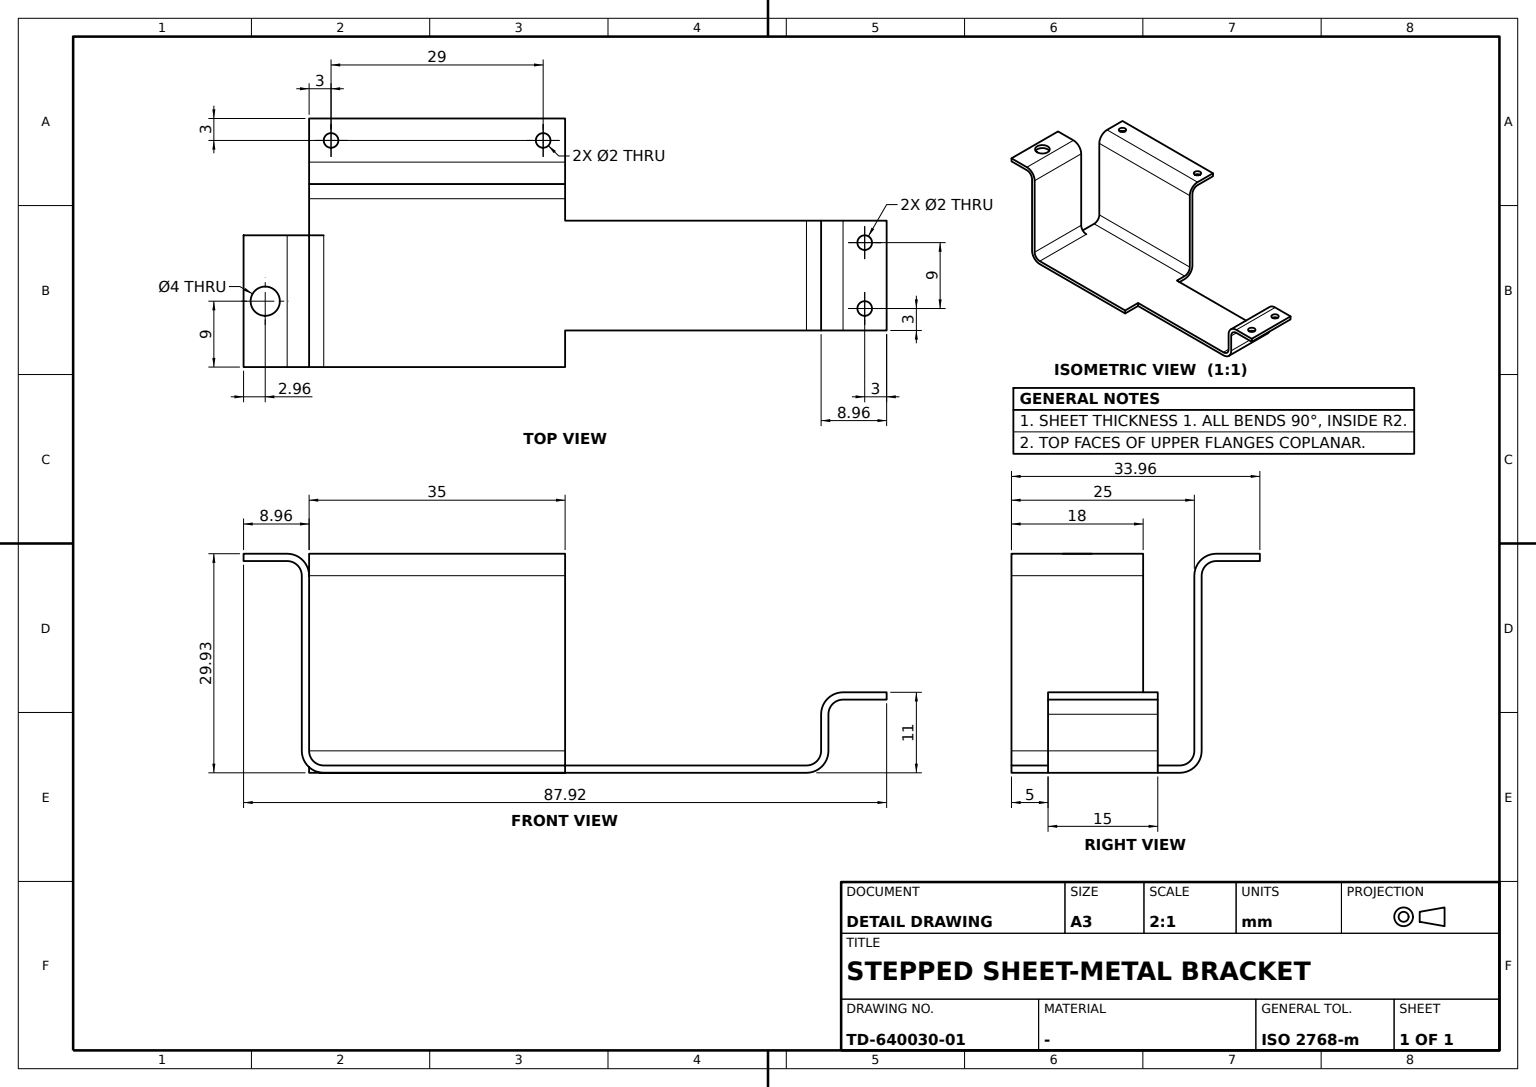
ISO-10303-21;
HEADER;
FILE_DESCRIPTION((''),'2;1');
FILE_NAME('','',(''),(''),'','','');
FILE_SCHEMA(('AUTOMOTIVE_DESIGN'));
ENDSEC;
DATA;
#1=APPLICATION_CONTEXT('');
#2=PRODUCT_CONTEXT('',#1,'mechanical');
#3=PRODUCT('','','',(#2));
#4=PRODUCT_DEFINITION_FORMATION('','',#3);
#5=PRODUCT_DEFINITION_CONTEXT('',#1,'design');
#6=PRODUCT_DEFINITION('','',#4,#5);
#7=PRODUCT_DEFINITION_SHAPE('','',#6);
#8=(LENGTH_UNIT()NAMED_UNIT(*)SI_UNIT(.MILLI.,.METRE.));
#9=(NAMED_UNIT(*)PLANE_ANGLE_UNIT()SI_UNIT($,.RADIAN.));
#10=(NAMED_UNIT(*)SI_UNIT($,.STERADIAN.)SOLID_ANGLE_UNIT());
#11=UNCERTAINTY_MEASURE_WITH_UNIT(LENGTH_MEASURE(0.005),#8,'distance_accuracy_value','');
#12=(GEOMETRIC_REPRESENTATION_CONTEXT(3)GLOBAL_UNCERTAINTY_ASSIGNED_CONTEXT((#11))GLOBAL_UNIT_ASSIGNED_CONTEXT((#8,#9,#10))REPRESENTATION_CONTEXT('',''));
#13=CARTESIAN_POINT('',(-5.5,-1.,3.));
#14=VERTEX_POINT('',#13);
#15=CARTESIAN_POINT('',(12.5,-1.,3.));
#16=VERTEX_POINT('',#15);
#17=CARTESIAN_POINT('',(1.,-1.,3.));
#18=DIRECTION('',(1.,0.,0.));
#19=VECTOR('',#18,1000.);
#20=LINE('',#17,#19);
#21=EDGE_CURVE('',#14,#16,#20,.T.);
#22=ORIENTED_EDGE('',*,*,#21,.F.);
#23=CARTESIAN_POINT('',(-5.5,2.,0.));
#24=VERTEX_POINT('',#23);
#25=CARTESIAN_POINT('',(-5.5,2.,3.));
#26=DIRECTION('',(-1.,0.,0.));
#27=DIRECTION('',(0.,0.,1.));
#28=AXIS2_PLACEMENT_3D('',#25,#26,#27);
#29=CIRCLE('',#28,3.);
#30=EDGE_CURVE('',#24,#14,#29,.T.);
#31=ORIENTED_EDGE('',*,*,#30,.F.);
#32=CARTESIAN_POINT('',(12.5,2.,0.));
#33=VERTEX_POINT('',#32);
#34=CARTESIAN_POINT('',(1.,2.,0.));
#35=LINE('',#34,#19);
#36=EDGE_CURVE('',#24,#33,#35,.T.);
#37=ORIENTED_EDGE('',*,*,#36,.T.);
#38=CARTESIAN_POINT('',(12.5,2.,3.));
#39=DIRECTION('',(0.,0.,-1.));
#40=AXIS2_PLACEMENT_3D('',#38,#18,#39);
#41=CIRCLE('',#40,3.);
#42=EDGE_CURVE('',#16,#33,#41,.T.);
#43=ORIENTED_EDGE('',*,*,#42,.F.);
#44=EDGE_LOOP('',(#22,#31,#37,#43));
#45=FACE_BOUND('',#44,.T.);
#46=CARTESIAN_POINT('',(1.,2.,3.));
#47=AXIS2_PLACEMENT_3D('',#46,#18,#39);
#48=CYLINDRICAL_SURFACE('',#47,3.);
#49=ADVANCED_FACE('',(#45),#48,.T.);
#50=CARTESIAN_POINT('',(7.5,73.,11.));
#51=VERTEX_POINT('',#50);
#52=CARTESIAN_POINT('',(-7.5,73.,11.));
#53=VERTEX_POINT('',#52);
#54=CARTESIAN_POINT('',(0.,73.,11.));
#55=VECTOR('',#26,1000.);
#56=LINE('',#54,#55);
#57=EDGE_CURVE('',#51,#53,#56,.T.);
#58=ORIENTED_EDGE('',*,*,#57,.F.);
#59=CARTESIAN_POINT('',(7.5,78.96,11.));
#60=VERTEX_POINT('',#59);
#61=CARTESIAN_POINT('',(7.5,35.,11.));
#62=DIRECTION('',(0.,-1.,0.));
#63=VECTOR('',#62,1000.);
#64=LINE('',#61,#63);
#65=EDGE_CURVE('',#51,#60,#64,.F.);
#66=ORIENTED_EDGE('',*,*,#65,.T.);
#67=CARTESIAN_POINT('',(-7.5,78.96,11.));
#68=VERTEX_POINT('',#67);
#69=CARTESIAN_POINT('',(0.,78.96,11.));
#70=LINE('',#69,#55);
#71=EDGE_CURVE('',#60,#68,#70,.T.);
#72=ORIENTED_EDGE('',*,*,#71,.T.);
#73=CARTESIAN_POINT('',(-7.5,71.,11.));
#74=LINE('',#73,#63);
#75=EDGE_CURVE('',#68,#53,#74,.T.);
#76=ORIENTED_EDGE('',*,*,#75,.T.);
#77=EDGE_LOOP('',(#58,#66,#72,#76));
#78=FACE_BOUND('',#77,.T.);
#79=CARTESIAN_POINT('',(-3.5,75.96,11.));
#80=VERTEX_POINT('',#79);
#81=CARTESIAN_POINT('',(-4.5,75.96,11.));
#82=AXIS2_PLACEMENT_3D('',#81,#27,#18);
#83=CIRCLE('',#82,1.);
#84=EDGE_CURVE('',#80,#80,#83,.T.);
#85=ORIENTED_EDGE('',*,*,#84,.F.);
#86=EDGE_LOOP('',(#85));
#87=FACE_BOUND('',#86,.T.);
#88=CARTESIAN_POINT('',(5.5,75.96,11.));
#89=VERTEX_POINT('',#88);
#90=CARTESIAN_POINT('',(4.5,75.96,11.));
#91=AXIS2_PLACEMENT_3D('',#90,#27,#18);
#92=CIRCLE('',#91,1.);
#93=EDGE_CURVE('',#89,#89,#92,.T.);
#94=ORIENTED_EDGE('',*,*,#93,.F.);
#95=EDGE_LOOP('',(#94));
#96=FACE_BOUND('',#95,.T.);
#97=CARTESIAN_POINT('',(0.,71.,11.));
#98=AXIS2_PLACEMENT_3D('',#97,#27,#18);
#99=PLANE('',#98);
#100=ADVANCED_FACE('',(#78,#87,#96),#99,.T.);
#101=CARTESIAN_POINT('',(-5.5,2.,1.));
#102=VERTEX_POINT('',#101);
#103=CARTESIAN_POINT('',(-5.5,0.,3.));
#104=VERTEX_POINT('',#103);
#105=CIRCLE('',#28,2.);
#106=EDGE_CURVE('',#102,#104,#105,.T.);
#107=ORIENTED_EDGE('',*,*,#106,.T.);
#108=CARTESIAN_POINT('',(12.5,0.,3.));
#109=VERTEX_POINT('',#108);
#110=CARTESIAN_POINT('',(1.,0.,3.));
#111=LINE('',#110,#19);
#112=EDGE_CURVE('',#104,#109,#111,.T.);
#113=ORIENTED_EDGE('',*,*,#112,.T.);
#114=CARTESIAN_POINT('',(12.5,2.,1.));
#115=VERTEX_POINT('',#114);
#116=CIRCLE('',#40,2.);
#117=EDGE_CURVE('',#109,#115,#116,.T.);
#118=ORIENTED_EDGE('',*,*,#117,.T.);
#119=CARTESIAN_POINT('',(1.,2.,1.));
#120=LINE('',#119,#19);
#121=EDGE_CURVE('',#102,#115,#120,.T.);
#122=ORIENTED_EDGE('',*,*,#121,.F.);
#123=EDGE_LOOP('',(#107,#113,#118,#122));
#124=FACE_BOUND('',#123,.T.);
#125=CYLINDRICAL_SURFACE('',#47,2.);
#126=ADVANCED_FACE('',(#124),#125,.F.);
#127=CARTESIAN_POINT('',(5.5,-6.,29.93));
#128=VERTEX_POINT('',#127);
#129=CARTESIAN_POINT('',(3.5,-6.,29.93));
#130=AXIS2_PLACEMENT_3D('',#129,#27,#18);
#131=CIRCLE('',#130,2.);
#132=EDGE_CURVE('',#128,#128,#131,.T.);
#133=ORIENTED_EDGE('',*,*,#132,.F.);
#134=EDGE_LOOP('',(#133));
#135=FACE_BOUND('',#134,.T.);
#136=CARTESIAN_POINT('',(12.5,-8.96,29.93));
#137=VERTEX_POINT('',#136);
#138=CARTESIAN_POINT('',(12.5,-3.,29.93));
#139=VERTEX_POINT('',#138);
#140=CARTESIAN_POINT('',(12.5,17.5,29.93));
#141=DIRECTION('',(0.,1.,0.));
#142=VECTOR('',#141,1000.);
#143=LINE('',#140,#142);
#144=EDGE_CURVE('',#137,#139,#143,.T.);
#145=ORIENTED_EDGE('',*,*,#144,.T.);
#146=CARTESIAN_POINT('',(-5.5,-3.,29.93));
#147=VERTEX_POINT('',#146);
#148=CARTESIAN_POINT('',(3.5,-3.,29.93));
#149=LINE('',#148,#19);
#150=EDGE_CURVE('',#147,#139,#149,.T.);
#151=ORIENTED_EDGE('',*,*,#150,.F.);
#152=CARTESIAN_POINT('',(-5.5,-8.96,29.93));
#153=VERTEX_POINT('',#152);
#154=CARTESIAN_POINT('',(-5.5,1.,29.93));
#155=LINE('',#154,#142);
#156=EDGE_CURVE('',#147,#153,#155,.F.);
#157=ORIENTED_EDGE('',*,*,#156,.T.);
#158=CARTESIAN_POINT('',(3.5,-8.96,29.93));
#159=LINE('',#158,#19);
#160=EDGE_CURVE('',#153,#137,#159,.T.);
#161=ORIENTED_EDGE('',*,*,#160,.T.);
#162=EDGE_LOOP('',(#145,#151,#157,#161));
#163=FACE_BOUND('',#162,.T.);
#164=CARTESIAN_POINT('',(-13.5,17.5,29.93));
#165=AXIS2_PLACEMENT_3D('',#164,#27,#141);
#166=PLANE('',#165);
#167=ADVANCED_FACE('',(#135,#163),#166,.T.);
#168=CARTESIAN_POINT('',(-15.5,0.,28.93));
#169=VERTEX_POINT('',#168);
#170=CARTESIAN_POINT('',(-15.5,35.,28.93));
#171=VERTEX_POINT('',#170);
#172=CARTESIAN_POINT('',(-15.5,17.5,28.93));
#173=LINE('',#172,#142);
#174=EDGE_CURVE('',#169,#171,#173,.T.);
#175=ORIENTED_EDGE('',*,*,#174,.T.);
#176=CARTESIAN_POINT('',(-13.5,35.,26.93));
#177=VERTEX_POINT('',#176);
#178=CARTESIAN_POINT('',(-15.5,35.,26.93));
#179=AXIS2_PLACEMENT_3D('',#178,#62,#39);
#180=CIRCLE('',#179,2.);
#181=EDGE_CURVE('',#171,#177,#180,.F.);
#182=ORIENTED_EDGE('',*,*,#181,.T.);
#183=CARTESIAN_POINT('',(-13.5,0.,26.93));
#184=VERTEX_POINT('',#183);
#185=CARTESIAN_POINT('',(-13.5,17.5,26.93));
#186=LINE('',#185,#142);
#187=EDGE_CURVE('',#184,#177,#186,.T.);
#188=ORIENTED_EDGE('',*,*,#187,.F.);
#189=CARTESIAN_POINT('',(-15.5,0.,26.93));
#190=AXIS2_PLACEMENT_3D('',#189,#62,#39);
#191=CIRCLE('',#190,2.);
#192=EDGE_CURVE('',#169,#184,#191,.F.);
#193=ORIENTED_EDGE('',*,*,#192,.F.);
#194=EDGE_LOOP('',(#175,#182,#188,#193));
#195=FACE_BOUND('',#194,.T.);
#196=CARTESIAN_POINT('',(-15.5,17.5,26.93));
#197=AXIS2_PLACEMENT_3D('',#196,#141,#18);
#198=CYLINDRICAL_SURFACE('',#197,2.);
#199=ADVANCED_FACE('',(#195),#198,.F.);
#200=CARTESIAN_POINT('',(-17.46,32.,28.93));
#201=VERTEX_POINT('',#200);
#202=CARTESIAN_POINT('',(-18.46,32.,28.93));
#203=AXIS2_PLACEMENT_3D('',#202,#27,#18);
#204=CIRCLE('',#203,1.);
#205=EDGE_CURVE('',#201,#201,#204,.T.);
#206=ORIENTED_EDGE('',*,*,#205,.T.);
#207=EDGE_LOOP('',(#206));
#208=FACE_BOUND('',#207,.T.);
#209=CARTESIAN_POINT('',(-21.46,0.,28.93));
#210=VERTEX_POINT('',#209);
#211=CARTESIAN_POINT('',(-13.5,0.,28.93));
#212=LINE('',#211,#19);
#213=EDGE_CURVE('',#210,#169,#212,.T.);
#214=ORIENTED_EDGE('',*,*,#213,.F.);
#215=CARTESIAN_POINT('',(-21.46,35.,28.93));
#216=VERTEX_POINT('',#215);
#217=CARTESIAN_POINT('',(-21.46,17.5,28.93));
#218=LINE('',#217,#63);
#219=EDGE_CURVE('',#216,#210,#218,.T.);
#220=ORIENTED_EDGE('',*,*,#219,.F.);
#221=CARTESIAN_POINT('',(-18.48,35.,28.93));
#222=LINE('',#221,#55);
#223=EDGE_CURVE('',#171,#216,#222,.T.);
#224=ORIENTED_EDGE('',*,*,#223,.F.);
#225=ORIENTED_EDGE('',*,*,#174,.F.);
#226=EDGE_LOOP('',(#214,#220,#224,#225));
#227=FACE_BOUND('',#226,.T.);
#228=CARTESIAN_POINT('',(-17.46,3.,28.93));
#229=VERTEX_POINT('',#228);
#230=CARTESIAN_POINT('',(-18.46,3.,28.93));
#231=AXIS2_PLACEMENT_3D('',#230,#27,#18);
#232=CIRCLE('',#231,1.);
#233=EDGE_CURVE('',#229,#229,#232,.T.);
#234=ORIENTED_EDGE('',*,*,#233,.T.);
#235=EDGE_LOOP('',(#234));
#236=FACE_BOUND('',#235,.T.);
#237=CARTESIAN_POINT('',(-13.5,17.5,28.93));
#238=AXIS2_PLACEMENT_3D('',#237,#27,#141);
#239=PLANE('',#238);
#240=ADVANCED_FACE('',(#208,#227,#236),#239,.F.);
#241=CARTESIAN_POINT('',(-21.46,35.,29.93));
#242=VERTEX_POINT('',#241);
#243=VECTOR('',#27,1000.);
#244=LINE('',#241,#243);
#245=EDGE_CURVE('',#216,#242,#244,.T.);
#246=ORIENTED_EDGE('',*,*,#245,.F.);
#247=ORIENTED_EDGE('',*,*,#219,.T.);
#248=CARTESIAN_POINT('',(-21.46,0.,29.93));
#249=VERTEX_POINT('',#248);
#250=LINE('',#248,#243);
#251=EDGE_CURVE('',#210,#249,#250,.T.);
#252=ORIENTED_EDGE('',*,*,#251,.T.);
#253=CARTESIAN_POINT('',(-21.46,17.5,29.93));
#254=LINE('',#253,#63);
#255=EDGE_CURVE('',#242,#249,#254,.T.);
#256=ORIENTED_EDGE('',*,*,#255,.F.);
#257=EDGE_LOOP('',(#246,#247,#252,#256));
#258=FACE_BOUND('',#257,.T.);
#259=AXIS2_PLACEMENT_3D('',#253,#18,#141);
#260=PLANE('',#259);
#261=ADVANCED_FACE('',(#258),#260,.F.);
#262=ORIENTED_EDGE('',*,*,#205,.F.);
#263=EDGE_LOOP('',(#262));
#264=FACE_BOUND('',#263,.T.);
#265=CARTESIAN_POINT('',(-17.46,32.,29.93));
#266=VERTEX_POINT('',#265);
#267=CARTESIAN_POINT('',(-18.46,32.,29.93));
#268=AXIS2_PLACEMENT_3D('',#267,#27,#18);
#269=CIRCLE('',#268,1.);
#270=EDGE_CURVE('',#266,#266,#269,.T.);
#271=ORIENTED_EDGE('',*,*,#270,.T.);
#272=EDGE_LOOP('',(#271));
#273=FACE_BOUND('',#272,.T.);
#274=CARTESIAN_POINT('',(-18.46,32.,29.43));
#275=AXIS2_PLACEMENT_3D('',#274,#39,#18);
#276=CYLINDRICAL_SURFACE('',#275,1.);
#277=ADVANCED_FACE('',(#264,#273),#276,.F.);
#278=CARTESIAN_POINT('',(7.5,68.,1.));
#279=VERTEX_POINT('',#278);
#280=CARTESIAN_POINT('',(-7.5,68.,1.));
#281=VERTEX_POINT('',#280);
#282=CARTESIAN_POINT('',(0.,68.,1.));
#283=LINE('',#282,#55);
#284=EDGE_CURVE('',#279,#281,#283,.T.);
#285=ORIENTED_EDGE('',*,*,#284,.T.);
#286=CARTESIAN_POINT('',(-7.5,35.,1.));
#287=VERTEX_POINT('',#286);
#288=CARTESIAN_POINT('',(-7.5,0.,1.));
#289=LINE('',#288,#63);
#290=EDGE_CURVE('',#281,#287,#289,.T.);
#291=ORIENTED_EDGE('',*,*,#290,.T.);
#292=CARTESIAN_POINT('',(-10.5,35.,1.));
#293=VERTEX_POINT('',#292);
#294=CARTESIAN_POINT('',(0.,35.,1.));
#295=LINE('',#294,#19);
#296=EDGE_CURVE('',#287,#293,#295,.F.);
#297=ORIENTED_EDGE('',*,*,#296,.T.);
#298=CARTESIAN_POINT('',(-10.5,0.,1.));
#299=VERTEX_POINT('',#298);
#300=CARTESIAN_POINT('',(-10.5,34.,1.));
#301=LINE('',#300,#63);
#302=EDGE_CURVE('',#293,#299,#301,.T.);
#303=ORIENTED_EDGE('',*,*,#302,.T.);
#304=CARTESIAN_POINT('',(-5.5,0.,1.));
#305=VERTEX_POINT('',#304);
#306=CARTESIAN_POINT('',(0.,0.,1.));
#307=LINE('',#306,#19);
#308=EDGE_CURVE('',#299,#305,#307,.T.);
#309=ORIENTED_EDGE('',*,*,#308,.T.);
#310=CARTESIAN_POINT('',(-5.5,1.,1.));
#311=LINE('',#310,#142);
#312=EDGE_CURVE('',#305,#102,#311,.T.);
#313=ORIENTED_EDGE('',*,*,#312,.T.);
#314=ORIENTED_EDGE('',*,*,#121,.T.);
#315=CARTESIAN_POINT('',(12.5,35.,1.));
#316=VERTEX_POINT('',#315);
#317=CARTESIAN_POINT('',(12.5,0.,1.));
#318=LINE('',#317,#142);
#319=EDGE_CURVE('',#115,#316,#318,.T.);
#320=ORIENTED_EDGE('',*,*,#319,.T.);
#321=CARTESIAN_POINT('',(7.5,35.,1.));
#322=VERTEX_POINT('',#321);
#323=EDGE_CURVE('',#316,#322,#295,.F.);
#324=ORIENTED_EDGE('',*,*,#323,.T.);
#325=CARTESIAN_POINT('',(7.5,0.,1.));
#326=LINE('',#325,#142);
#327=EDGE_CURVE('',#322,#279,#326,.T.);
#328=ORIENTED_EDGE('',*,*,#327,.T.);
#329=EDGE_LOOP('',(#285,#291,#297,#303,#309,#313,#314,#320,#324,#328));
#330=FACE_BOUND('',#329,.T.);
#331=AXIS2_PLACEMENT_3D('',#306,#27,#141);
#332=PLANE('',#331);
#333=ADVANCED_FACE('',(#330),#332,.T.);
#334=ORIENTED_EDGE('',*,*,#30,.T.);
#335=CARTESIAN_POINT('',(-5.5,-1.,26.93));
#336=VERTEX_POINT('',#335);
#337=CARTESIAN_POINT('',(-5.5,-1.,1.));
#338=VECTOR('',#39,1000.);
#339=LINE('',#337,#338);
#340=EDGE_CURVE('',#336,#14,#339,.T.);
#341=ORIENTED_EDGE('',*,*,#340,.F.);
#342=CARTESIAN_POINT('',(-5.5,-3.,28.93));
#343=VERTEX_POINT('',#342);
#344=CARTESIAN_POINT('',(-5.5,-3.,26.93));
#345=AXIS2_PLACEMENT_3D('',#344,#26,#27);
#346=CIRCLE('',#345,2.);
#347=EDGE_CURVE('',#343,#336,#346,.T.);
#348=ORIENTED_EDGE('',*,*,#347,.F.);
#349=CARTESIAN_POINT('',(-5.5,-8.96,28.93));
#350=VERTEX_POINT('',#349);
#351=CARTESIAN_POINT('',(-5.5,1.,28.93));
#352=LINE('',#351,#142);
#353=EDGE_CURVE('',#343,#350,#352,.F.);
#354=ORIENTED_EDGE('',*,*,#353,.T.);
#355=CARTESIAN_POINT('',(-5.5,-8.96,0.));
#356=LINE('',#355,#338);
#357=EDGE_CURVE('',#350,#153,#356,.F.);
#358=ORIENTED_EDGE('',*,*,#357,.T.);
#359=ORIENTED_EDGE('',*,*,#156,.F.);
#360=CARTESIAN_POINT('',(-5.5,0.,26.93));
#361=VERTEX_POINT('',#360);
#362=CIRCLE('',#345,3.);
#363=EDGE_CURVE('',#147,#361,#362,.T.);
#364=ORIENTED_EDGE('',*,*,#363,.T.);
#365=CARTESIAN_POINT('',(-5.5,0.,0.));
#366=LINE('',#365,#243);
#367=EDGE_CURVE('',#104,#361,#366,.T.);
#368=ORIENTED_EDGE('',*,*,#367,.F.);
#369=ORIENTED_EDGE('',*,*,#106,.F.);
#370=LINE('',#23,#338);
#371=EDGE_CURVE('',#24,#102,#370,.F.);
#372=ORIENTED_EDGE('',*,*,#371,.F.);
#373=EDGE_LOOP('',(#334,#341,#348,#354,#358,#359,#364,#368,#369,#372));
#374=FACE_BOUND('',#373,.T.);
#375=CARTESIAN_POINT('',(-5.5,1.,0.));
#376=AXIS2_PLACEMENT_3D('',#375,#26,#141);
#377=PLANE('',#376);
#378=ADVANCED_FACE('',(#374),#377,.T.);
#379=ORIENTED_EDGE('',*,*,#93,.T.);
#380=EDGE_LOOP('',(#379));
#381=FACE_BOUND('',#380,.T.);
#382=CARTESIAN_POINT('',(5.5,75.96,10.));
#383=VERTEX_POINT('',#382);
#384=CARTESIAN_POINT('',(4.5,75.96,10.));
#385=AXIS2_PLACEMENT_3D('',#384,#27,#18);
#386=CIRCLE('',#385,1.);
#387=EDGE_CURVE('',#383,#383,#386,.T.);
#388=ORIENTED_EDGE('',*,*,#387,.F.);
#389=EDGE_LOOP('',(#388));
#390=FACE_BOUND('',#389,.T.);
#391=CARTESIAN_POINT('',(4.5,75.96,10.5));
#392=AXIS2_PLACEMENT_3D('',#391,#39,#18);
#393=CYLINDRICAL_SURFACE('',#392,1.);
#394=ADVANCED_FACE('',(#381,#390),#393,.F.);
#395=ORIENTED_EDGE('',*,*,#245,.T.);
#396=CARTESIAN_POINT('',(-15.5,35.,29.93));
#397=VERTEX_POINT('',#396);
#398=CARTESIAN_POINT('',(-18.48,35.,29.93));
#399=LINE('',#398,#55);
#400=EDGE_CURVE('',#397,#242,#399,.T.);
#401=ORIENTED_EDGE('',*,*,#400,.F.);
#402=CARTESIAN_POINT('',(-12.5,35.,26.93));
#403=VERTEX_POINT('',#402);
#404=CIRCLE('',#179,3.);
#405=EDGE_CURVE('',#397,#403,#404,.F.);
#406=ORIENTED_EDGE('',*,*,#405,.T.);
#407=CARTESIAN_POINT('',(-12.5,35.,3.));
#408=VERTEX_POINT('',#407);
#409=CARTESIAN_POINT('',(-12.5,35.,29.93));
#410=LINE('',#409,#338);
#411=EDGE_CURVE('',#408,#403,#410,.F.);
#412=ORIENTED_EDGE('',*,*,#411,.F.);
#413=CARTESIAN_POINT('',(-10.5,35.,3.));
#414=AXIS2_PLACEMENT_3D('',#413,#62,#39);
#415=CIRCLE('',#414,2.);
#416=EDGE_CURVE('',#408,#293,#415,.T.);
#417=ORIENTED_EDGE('',*,*,#416,.T.);
#418=ORIENTED_EDGE('',*,*,#296,.F.);
#419=CARTESIAN_POINT('',(-7.5,35.,0.));
#420=VERTEX_POINT('',#419);
#421=LINE('',#419,#243);
#422=EDGE_CURVE('',#287,#420,#421,.F.);
#423=ORIENTED_EDGE('',*,*,#422,.T.);
#424=CARTESIAN_POINT('',(-10.5,35.,0.));
#425=VERTEX_POINT('',#424);
#426=CARTESIAN_POINT('',(0.,35.,0.));
#427=LINE('',#426,#19);
#428=EDGE_CURVE('',#420,#425,#427,.F.);
#429=ORIENTED_EDGE('',*,*,#428,.T.);
#430=CARTESIAN_POINT('',(-13.5,35.,3.));
#431=VERTEX_POINT('',#430);
#432=CIRCLE('',#414,3.);
#433=EDGE_CURVE('',#431,#425,#432,.T.);
#434=ORIENTED_EDGE('',*,*,#433,.F.);
#435=CARTESIAN_POINT('',(-13.5,35.,1.));
#436=LINE('',#435,#243);
#437=EDGE_CURVE('',#177,#431,#436,.F.);
#438=ORIENTED_EDGE('',*,*,#437,.F.);
#439=ORIENTED_EDGE('',*,*,#181,.F.);
#440=ORIENTED_EDGE('',*,*,#223,.T.);
#441=EDGE_LOOP('',(#395,#401,#406,#412,#417,#418,#423,#429,#434,#438,#439,#440));
#442=FACE_BOUND('',#441,.T.);
#443=AXIS2_PLACEMENT_3D('',#398,#62,#18);
#444=PLANE('',#443);
#445=ADVANCED_FACE('',(#442),#444,.F.);
#446=CARTESIAN_POINT('',(-12.5,0.,3.));
#447=VERTEX_POINT('',#446);
#448=CARTESIAN_POINT('',(-10.5,0.,3.));
#449=AXIS2_PLACEMENT_3D('',#448,#62,#39);
#450=CIRCLE('',#449,2.);
#451=EDGE_CURVE('',#447,#299,#450,.T.);
#452=ORIENTED_EDGE('',*,*,#451,.F.);
#453=CARTESIAN_POINT('',(-12.5,0.,26.93));
#454=VERTEX_POINT('',#453);
#455=CARTESIAN_POINT('',(-12.5,0.,29.93));
#456=LINE('',#455,#338);
#457=EDGE_CURVE('',#447,#454,#456,.F.);
#458=ORIENTED_EDGE('',*,*,#457,.T.);
#459=CARTESIAN_POINT('',(-15.5,0.,29.93));
#460=VERTEX_POINT('',#459);
#461=CIRCLE('',#190,3.);
#462=EDGE_CURVE('',#460,#454,#461,.F.);
#463=ORIENTED_EDGE('',*,*,#462,.F.);
#464=CARTESIAN_POINT('',(-13.5,0.,29.93));
#465=LINE('',#464,#19);
#466=EDGE_CURVE('',#249,#460,#465,.T.);
#467=ORIENTED_EDGE('',*,*,#466,.F.);
#468=ORIENTED_EDGE('',*,*,#251,.F.);
#469=ORIENTED_EDGE('',*,*,#213,.T.);
#470=ORIENTED_EDGE('',*,*,#192,.T.);
#471=CARTESIAN_POINT('',(-13.5,0.,3.));
#472=VERTEX_POINT('',#471);
#473=CARTESIAN_POINT('',(-13.5,0.,1.));
#474=LINE('',#473,#243);
#475=EDGE_CURVE('',#184,#472,#474,.F.);
#476=ORIENTED_EDGE('',*,*,#475,.T.);
#477=CARTESIAN_POINT('',(-10.5,0.,0.));
#478=VERTEX_POINT('',#477);
#479=CIRCLE('',#449,3.);
#480=EDGE_CURVE('',#472,#478,#479,.T.);
#481=ORIENTED_EDGE('',*,*,#480,.T.);
#482=VERTEX_POINT('',#365);
#483=CARTESIAN_POINT('',(0.,0.,0.));
#484=LINE('',#483,#19);
#485=EDGE_CURVE('',#478,#482,#484,.T.);
#486=ORIENTED_EDGE('',*,*,#485,.T.);
#487=EDGE_CURVE('',#482,#305,#366,.T.);
#488=ORIENTED_EDGE('',*,*,#487,.T.);
#489=ORIENTED_EDGE('',*,*,#308,.F.);
#490=EDGE_LOOP('',(#452,#458,#463,#467,#468,#469,#470,#476,#481,#486,#488,#489));
#491=FACE_BOUND('',#490,.T.);
#492=CARTESIAN_POINT('',(-18.48,0.,29.93));
#493=AXIS2_PLACEMENT_3D('',#492,#62,#18);
#494=PLANE('',#493);
#495=ADVANCED_FACE('',(#491),#494,.T.);
#496=CARTESIAN_POINT('',(7.5,73.,10.));
#497=VERTEX_POINT('',#496);
#498=CARTESIAN_POINT('',(7.5,71.,8.));
#499=VERTEX_POINT('',#498);
#500=CARTESIAN_POINT('',(7.5,73.,8.));
#501=AXIS2_PLACEMENT_3D('',#500,#18,#39);
#502=CIRCLE('',#501,2.);
#503=EDGE_CURVE('',#497,#499,#502,.T.);
#504=ORIENTED_EDGE('',*,*,#503,.T.);
#505=CARTESIAN_POINT('',(-7.5,71.,8.));
#506=VERTEX_POINT('',#505);
#507=CARTESIAN_POINT('',(0.,71.,8.));
#508=LINE('',#507,#55);
#509=EDGE_CURVE('',#499,#506,#508,.T.);
#510=ORIENTED_EDGE('',*,*,#509,.T.);
#511=CARTESIAN_POINT('',(-7.5,73.,10.));
#512=VERTEX_POINT('',#511);
#513=CARTESIAN_POINT('',(-7.5,73.,8.));
#514=AXIS2_PLACEMENT_3D('',#513,#26,#27);
#515=CIRCLE('',#514,2.);
#516=EDGE_CURVE('',#512,#506,#515,.F.);
#517=ORIENTED_EDGE('',*,*,#516,.F.);
#518=CARTESIAN_POINT('',(0.,73.,10.));
#519=LINE('',#518,#55);
#520=EDGE_CURVE('',#497,#512,#519,.T.);
#521=ORIENTED_EDGE('',*,*,#520,.F.);
#522=EDGE_LOOP('',(#504,#510,#517,#521));
#523=FACE_BOUND('',#522,.T.);
#524=CARTESIAN_POINT('',(0.,73.,8.));
#525=AXIS2_PLACEMENT_3D('',#524,#26,#62);
#526=CYLINDRICAL_SURFACE('',#525,2.);
#527=ADVANCED_FACE('',(#523),#526,.F.);
#528=CARTESIAN_POINT('',(-3.5,75.96,10.));
#529=VERTEX_POINT('',#528);
#530=CARTESIAN_POINT('',(-4.5,75.96,10.));
#531=AXIS2_PLACEMENT_3D('',#530,#27,#18);
#532=CIRCLE('',#531,1.);
#533=EDGE_CURVE('',#529,#529,#532,.T.);
#534=ORIENTED_EDGE('',*,*,#533,.F.);
#535=EDGE_LOOP('',(#534));
#536=FACE_BOUND('',#535,.T.);
#537=ORIENTED_EDGE('',*,*,#84,.T.);
#538=EDGE_LOOP('',(#537));
#539=FACE_BOUND('',#538,.T.);
#540=CARTESIAN_POINT('',(-4.5,75.96,10.5));
#541=AXIS2_PLACEMENT_3D('',#540,#27,#26);
#542=CYLINDRICAL_SURFACE('',#541,1.);
#543=ADVANCED_FACE('',(#536,#539),#542,.F.);
#544=CARTESIAN_POINT('',(12.5,35.,0.));
#545=VERTEX_POINT('',#544);
#546=CARTESIAN_POINT('',(12.5,0.,0.));
#547=LINE('',#546,#142);
#548=EDGE_CURVE('',#33,#545,#547,.T.);
#549=ORIENTED_EDGE('',*,*,#548,.T.);
#550=CARTESIAN_POINT('',(12.5,35.,29.93));
#551=LINE('',#550,#243);
#552=EDGE_CURVE('',#316,#545,#551,.F.);
#553=ORIENTED_EDGE('',*,*,#552,.F.);
#554=ORIENTED_EDGE('',*,*,#319,.F.);
#555=ORIENTED_EDGE('',*,*,#117,.F.);
#556=CARTESIAN_POINT('',(12.5,0.,26.93));
#557=VERTEX_POINT('',#556);
#558=LINE('',#546,#338);
#559=EDGE_CURVE('',#109,#557,#558,.F.);
#560=ORIENTED_EDGE('',*,*,#559,.T.);
#561=CARTESIAN_POINT('',(12.5,-3.,26.93));
#562=AXIS2_PLACEMENT_3D('',#561,#18,#39);
#563=CIRCLE('',#562,3.);
#564=EDGE_CURVE('',#139,#557,#563,.F.);
#565=ORIENTED_EDGE('',*,*,#564,.F.);
#566=ORIENTED_EDGE('',*,*,#144,.F.);
#567=CARTESIAN_POINT('',(12.5,-8.96,28.93));
#568=VERTEX_POINT('',#567);
#569=CARTESIAN_POINT('',(12.5,-8.96,0.));
#570=LINE('',#569,#243);
#571=EDGE_CURVE('',#568,#137,#570,.T.);
#572=ORIENTED_EDGE('',*,*,#571,.F.);
#573=CARTESIAN_POINT('',(12.5,-3.,28.93));
#574=VERTEX_POINT('',#573);
#575=CARTESIAN_POINT('',(12.5,17.5,28.93));
#576=LINE('',#575,#142);
#577=EDGE_CURVE('',#568,#574,#576,.T.);
#578=ORIENTED_EDGE('',*,*,#577,.T.);
#579=CARTESIAN_POINT('',(12.5,-1.,26.93));
#580=VERTEX_POINT('',#579);
#581=CIRCLE('',#562,2.);
#582=EDGE_CURVE('',#574,#580,#581,.F.);
#583=ORIENTED_EDGE('',*,*,#582,.T.);
#584=CARTESIAN_POINT('',(12.5,-1.,1.));
#585=LINE('',#584,#243);
#586=EDGE_CURVE('',#580,#16,#585,.F.);
#587=ORIENTED_EDGE('',*,*,#586,.T.);
#588=ORIENTED_EDGE('',*,*,#42,.T.);
#589=EDGE_LOOP('',(#549,#553,#554,#555,#560,#565,#566,#572,#578,#583,#587,#588));
#590=FACE_BOUND('',#589,.T.);
#591=AXIS2_PLACEMENT_3D('',#546,#18,#141);
#592=PLANE('',#591);
#593=ADVANCED_FACE('',(#590),#592,.T.);
#594=CARTESIAN_POINT('',(-7.5,71.,3.));
#595=VERTEX_POINT('',#594);
#596=CARTESIAN_POINT('',(-7.5,71.,1.));
#597=LINE('',#596,#243);
#598=EDGE_CURVE('',#506,#595,#597,.F.);
#599=ORIENTED_EDGE('',*,*,#598,.F.);
#600=ORIENTED_EDGE('',*,*,#509,.F.);
#601=CARTESIAN_POINT('',(7.5,71.,3.));
#602=VERTEX_POINT('',#601);
#603=CARTESIAN_POINT('',(7.5,71.,1.));
#604=LINE('',#603,#338);
#605=EDGE_CURVE('',#499,#602,#604,.T.);
#606=ORIENTED_EDGE('',*,*,#605,.T.);
#607=CARTESIAN_POINT('',(0.,71.,3.));
#608=LINE('',#607,#55);
#609=EDGE_CURVE('',#602,#595,#608,.T.);
#610=ORIENTED_EDGE('',*,*,#609,.T.);
#611=EDGE_LOOP('',(#599,#600,#606,#610));
#612=FACE_BOUND('',#611,.T.);
#613=CARTESIAN_POINT('',(0.,71.,1.));
#614=AXIS2_PLACEMENT_3D('',#613,#141,#26);
#615=PLANE('',#614);
#616=ADVANCED_FACE('',(#612),#615,.T.);
#617=ORIENTED_EDGE('',*,*,#357,.F.);
#618=CARTESIAN_POINT('',(3.5,-8.96,28.93));
#619=LINE('',#618,#19);
#620=EDGE_CURVE('',#350,#568,#619,.T.);
#621=ORIENTED_EDGE('',*,*,#620,.T.);
#622=ORIENTED_EDGE('',*,*,#571,.T.);
#623=ORIENTED_EDGE('',*,*,#160,.F.);
#624=EDGE_LOOP('',(#617,#621,#622,#623));
#625=FACE_BOUND('',#624,.T.);
#626=AXIS2_PLACEMENT_3D('',#158,#141,#18);
#627=PLANE('',#626);
#628=ADVANCED_FACE('',(#625),#627,.F.);
#629=ORIENTED_EDGE('',*,*,#290,.F.);
#630=CARTESIAN_POINT('',(-7.5,70.,3.));
#631=VERTEX_POINT('',#630);
#632=CARTESIAN_POINT('',(-7.5,68.,3.));
#633=AXIS2_PLACEMENT_3D('',#632,#26,#27);
#634=CIRCLE('',#633,2.);
#635=EDGE_CURVE('',#631,#281,#634,.T.);
#636=ORIENTED_EDGE('',*,*,#635,.F.);
#637=CARTESIAN_POINT('',(-7.5,70.,8.));
#638=VERTEX_POINT('',#637);
#639=CARTESIAN_POINT('',(-7.5,70.,0.));
#640=LINE('',#639,#338);
#641=EDGE_CURVE('',#631,#638,#640,.F.);
#642=ORIENTED_EDGE('',*,*,#641,.T.);
#643=CIRCLE('',#514,3.);
#644=EDGE_CURVE('',#53,#638,#643,.F.);
#645=ORIENTED_EDGE('',*,*,#644,.F.);
#646=ORIENTED_EDGE('',*,*,#75,.F.);
#647=CARTESIAN_POINT('',(-7.5,78.96,10.));
#648=VERTEX_POINT('',#647);
#649=CARTESIAN_POINT('',(-7.5,78.96,0.));
#650=LINE('',#649,#243);
#651=EDGE_CURVE('',#648,#68,#650,.T.);
#652=ORIENTED_EDGE('',*,*,#651,.F.);
#653=CARTESIAN_POINT('',(-7.5,71.,10.));
#654=LINE('',#653,#63);
#655=EDGE_CURVE('',#648,#512,#654,.T.);
#656=ORIENTED_EDGE('',*,*,#655,.T.);
#657=ORIENTED_EDGE('',*,*,#516,.T.);
#658=ORIENTED_EDGE('',*,*,#598,.T.);
#659=CARTESIAN_POINT('',(-7.5,68.,0.));
#660=VERTEX_POINT('',#659);
#661=CIRCLE('',#633,3.);
#662=EDGE_CURVE('',#595,#660,#661,.T.);
#663=ORIENTED_EDGE('',*,*,#662,.T.);
#664=CARTESIAN_POINT('',(-7.5,0.,0.));
#665=LINE('',#664,#63);
#666=EDGE_CURVE('',#660,#420,#665,.T.);
#667=ORIENTED_EDGE('',*,*,#666,.T.);
#668=ORIENTED_EDGE('',*,*,#422,.F.);
#669=EDGE_LOOP('',(#629,#636,#642,#645,#646,#652,#656,#657,#658,#663,#667,#668));
#670=FACE_BOUND('',#669,.T.);
#671=AXIS2_PLACEMENT_3D('',#639,#26,#62);
#672=PLANE('',#671);
#673=ADVANCED_FACE('',(#670),#672,.T.);
#674=CARTESIAN_POINT('',(-10.5,34.,0.));
#675=LINE('',#674,#63);
#676=EDGE_CURVE('',#425,#478,#675,.T.);
#677=ORIENTED_EDGE('',*,*,#676,.T.);
#678=ORIENTED_EDGE('',*,*,#480,.F.);
#679=CARTESIAN_POINT('',(-13.5,34.,3.));
#680=LINE('',#679,#63);
#681=EDGE_CURVE('',#431,#472,#680,.T.);
#682=ORIENTED_EDGE('',*,*,#681,.F.);
#683=ORIENTED_EDGE('',*,*,#433,.T.);
#684=EDGE_LOOP('',(#677,#678,#682,#683));
#685=FACE_BOUND('',#684,.T.);
#686=CARTESIAN_POINT('',(-10.5,34.,3.));
#687=AXIS2_PLACEMENT_3D('',#686,#62,#39);
#688=CYLINDRICAL_SURFACE('',#687,3.);
#689=ADVANCED_FACE('',(#685),#688,.T.);
#690=ORIENTED_EDGE('',*,*,#132,.T.);
#691=EDGE_LOOP('',(#690));
#692=FACE_BOUND('',#691,.T.);
#693=CARTESIAN_POINT('',(5.5,-6.,28.93));
#694=VERTEX_POINT('',#693);
#695=CARTESIAN_POINT('',(3.5,-6.,28.93));
#696=AXIS2_PLACEMENT_3D('',#695,#27,#18);
#697=CIRCLE('',#696,2.);
#698=EDGE_CURVE('',#694,#694,#697,.T.);
#699=ORIENTED_EDGE('',*,*,#698,.F.);
#700=EDGE_LOOP('',(#699));
#701=FACE_BOUND('',#700,.T.);
#702=CARTESIAN_POINT('',(3.5,-6.,29.43));
#703=AXIS2_PLACEMENT_3D('',#702,#39,#18);
#704=CYLINDRICAL_SURFACE('',#703,2.);
#705=ADVANCED_FACE('',(#692,#701),#704,.F.);
#706=ORIENTED_EDGE('',*,*,#371,.T.);
#707=ORIENTED_EDGE('',*,*,#312,.F.);
#708=ORIENTED_EDGE('',*,*,#487,.F.);
#709=LINE('',#375,#142);
#710=EDGE_CURVE('',#482,#24,#709,.T.);
#711=ORIENTED_EDGE('',*,*,#710,.T.);
#712=EDGE_LOOP('',(#706,#707,#708,#711));
#713=FACE_BOUND('',#712,.T.);
#714=ADVANCED_FACE('',(#713),#377,.F.);
#715=CARTESIAN_POINT('',(7.5,35.,0.));
#716=VERTEX_POINT('',#715);
#717=EDGE_CURVE('',#545,#716,#427,.F.);
#718=ORIENTED_EDGE('',*,*,#717,.T.);
#719=CARTESIAN_POINT('',(7.5,35.,29.93));
#720=LINE('',#719,#243);
#721=EDGE_CURVE('',#322,#716,#720,.F.);
#722=ORIENTED_EDGE('',*,*,#721,.F.);
#723=ORIENTED_EDGE('',*,*,#323,.F.);
#724=ORIENTED_EDGE('',*,*,#552,.T.);
#725=EDGE_LOOP('',(#718,#722,#723,#724));
#726=FACE_BOUND('',#725,.T.);
#727=ADVANCED_FACE('',(#726),#444,.F.);
#728=CARTESIAN_POINT('',(7.5,70.,3.));
#729=VERTEX_POINT('',#728);
#730=CARTESIAN_POINT('',(7.5,68.,3.));
#731=AXIS2_PLACEMENT_3D('',#730,#18,#39);
#732=CIRCLE('',#731,2.);
#733=EDGE_CURVE('',#729,#279,#732,.F.);
#734=ORIENTED_EDGE('',*,*,#733,.F.);
#735=CARTESIAN_POINT('',(0.,70.,3.));
#736=LINE('',#735,#55);
#737=EDGE_CURVE('',#729,#631,#736,.T.);
#738=ORIENTED_EDGE('',*,*,#737,.T.);
#739=ORIENTED_EDGE('',*,*,#635,.T.);
#740=ORIENTED_EDGE('',*,*,#284,.F.);
#741=EDGE_LOOP('',(#734,#738,#739,#740));
#742=FACE_BOUND('',#741,.T.);
#743=CARTESIAN_POINT('',(0.,68.,3.));
#744=AXIS2_PLACEMENT_3D('',#743,#26,#39);
#745=CYLINDRICAL_SURFACE('',#744,2.);
#746=ADVANCED_FACE('',(#742),#745,.F.);
#747=ORIENTED_EDGE('',*,*,#737,.F.);
#748=CARTESIAN_POINT('',(7.5,70.,8.));
#749=VERTEX_POINT('',#748);
#750=CARTESIAN_POINT('',(7.5,70.,0.));
#751=LINE('',#750,#243);
#752=EDGE_CURVE('',#729,#749,#751,.T.);
#753=ORIENTED_EDGE('',*,*,#752,.T.);
#754=CARTESIAN_POINT('',(0.,70.,8.));
#755=LINE('',#754,#55);
#756=EDGE_CURVE('',#749,#638,#755,.T.);
#757=ORIENTED_EDGE('',*,*,#756,.T.);
#758=ORIENTED_EDGE('',*,*,#641,.F.);
#759=EDGE_LOOP('',(#747,#753,#757,#758));
#760=FACE_BOUND('',#759,.T.);
#761=CARTESIAN_POINT('',(0.,70.,1.));
#762=AXIS2_PLACEMENT_3D('',#761,#141,#26);
#763=PLANE('',#762);
#764=ADVANCED_FACE('',(#760),#763,.F.);
#765=ORIENTED_EDGE('',*,*,#582,.F.);
#766=CARTESIAN_POINT('',(3.5,-3.,28.93));
#767=LINE('',#766,#19);
#768=EDGE_CURVE('',#343,#574,#767,.T.);
#769=ORIENTED_EDGE('',*,*,#768,.F.);
#770=ORIENTED_EDGE('',*,*,#347,.T.);
#771=CARTESIAN_POINT('',(3.5,-1.,26.93));
#772=LINE('',#771,#19);
#773=EDGE_CURVE('',#336,#580,#772,.T.);
#774=ORIENTED_EDGE('',*,*,#773,.T.);
#775=EDGE_LOOP('',(#765,#769,#770,#774));
#776=FACE_BOUND('',#775,.T.);
#777=CARTESIAN_POINT('',(3.5,-3.,26.93));
#778=AXIS2_PLACEMENT_3D('',#777,#18,#141);
#779=CYLINDRICAL_SURFACE('',#778,2.);
#780=ADVANCED_FACE('',(#776),#779,.F.);
#781=ORIENTED_EDGE('',*,*,#756,.F.);
#782=CIRCLE('',#501,3.);
#783=EDGE_CURVE('',#51,#749,#782,.T.);
#784=ORIENTED_EDGE('',*,*,#783,.F.);
#785=ORIENTED_EDGE('',*,*,#57,.T.);
#786=ORIENTED_EDGE('',*,*,#644,.T.);
#787=EDGE_LOOP('',(#781,#784,#785,#786));
#788=FACE_BOUND('',#787,.T.);
#789=CYLINDRICAL_SURFACE('',#525,3.);
#790=ADVANCED_FACE('',(#788),#789,.T.);
#791=CARTESIAN_POINT('',(-17.46,3.,29.93));
#792=VERTEX_POINT('',#791);
#793=CARTESIAN_POINT('',(-18.46,3.,29.93));
#794=AXIS2_PLACEMENT_3D('',#793,#27,#18);
#795=CIRCLE('',#794,1.);
#796=EDGE_CURVE('',#792,#792,#795,.T.);
#797=ORIENTED_EDGE('',*,*,#796,.F.);
#798=EDGE_LOOP('',(#797));
#799=FACE_BOUND('',#798,.T.);
#800=ORIENTED_EDGE('',*,*,#270,.F.);
#801=EDGE_LOOP('',(#800));
#802=FACE_BOUND('',#801,.T.);
#803=CARTESIAN_POINT('',(-15.5,17.5,29.93));
#804=LINE('',#803,#142);
#805=EDGE_CURVE('',#460,#397,#804,.T.);
#806=ORIENTED_EDGE('',*,*,#805,.T.);
#807=ORIENTED_EDGE('',*,*,#400,.T.);
#808=ORIENTED_EDGE('',*,*,#255,.T.);
#809=ORIENTED_EDGE('',*,*,#466,.T.);
#810=EDGE_LOOP('',(#806,#807,#808,#809));
#811=FACE_BOUND('',#810,.T.);
#812=ADVANCED_FACE('',(#799,#802,#811),#166,.T.);
#813=ORIENTED_EDGE('',*,*,#233,.F.);
#814=EDGE_LOOP('',(#813));
#815=FACE_BOUND('',#814,.T.);
#816=ORIENTED_EDGE('',*,*,#796,.T.);
#817=EDGE_LOOP('',(#816));
#818=FACE_BOUND('',#817,.T.);
#819=CARTESIAN_POINT('',(-18.46,3.,29.43));
#820=AXIS2_PLACEMENT_3D('',#819,#39,#18);
#821=CYLINDRICAL_SURFACE('',#820,1.);
#822=ADVANCED_FACE('',(#815,#818),#821,.F.);
#823=CARTESIAN_POINT('',(-12.5,17.5,26.93));
#824=LINE('',#823,#142);
#825=EDGE_CURVE('',#454,#403,#824,.T.);
#826=ORIENTED_EDGE('',*,*,#825,.T.);
#827=ORIENTED_EDGE('',*,*,#405,.F.);
#828=ORIENTED_EDGE('',*,*,#805,.F.);
#829=ORIENTED_EDGE('',*,*,#462,.T.);
#830=EDGE_LOOP('',(#826,#827,#828,#829));
#831=FACE_BOUND('',#830,.T.);
#832=CYLINDRICAL_SURFACE('',#197,3.);
#833=ADVANCED_FACE('',(#831),#832,.T.);
#834=ORIENTED_EDGE('',*,*,#533,.T.);
#835=EDGE_LOOP('',(#834));
#836=FACE_BOUND('',#835,.T.);
#837=ORIENTED_EDGE('',*,*,#655,.F.);
#838=CARTESIAN_POINT('',(7.5,78.96,10.));
#839=VERTEX_POINT('',#838);
#840=CARTESIAN_POINT('',(0.,78.96,10.));
#841=LINE('',#840,#55);
#842=EDGE_CURVE('',#839,#648,#841,.T.);
#843=ORIENTED_EDGE('',*,*,#842,.F.);
#844=CARTESIAN_POINT('',(7.5,35.,10.));
#845=LINE('',#844,#63);
#846=EDGE_CURVE('',#497,#839,#845,.F.);
#847=ORIENTED_EDGE('',*,*,#846,.F.);
#848=ORIENTED_EDGE('',*,*,#520,.T.);
#849=EDGE_LOOP('',(#837,#843,#847,#848));
#850=FACE_BOUND('',#849,.T.);
#851=ORIENTED_EDGE('',*,*,#387,.T.);
#852=EDGE_LOOP('',(#851));
#853=FACE_BOUND('',#852,.T.);
#854=CARTESIAN_POINT('',(0.,71.,10.));
#855=AXIS2_PLACEMENT_3D('',#854,#27,#18);
#856=PLANE('',#855);
#857=ADVANCED_FACE('',(#836,#850,#853),#856,.F.);
#858=ORIENTED_EDGE('',*,*,#564,.T.);
#859=CARTESIAN_POINT('',(3.5,0.,26.93));
#860=LINE('',#859,#19);
#861=EDGE_CURVE('',#361,#557,#860,.T.);
#862=ORIENTED_EDGE('',*,*,#861,.F.);
#863=ORIENTED_EDGE('',*,*,#363,.F.);
#864=ORIENTED_EDGE('',*,*,#150,.T.);
#865=EDGE_LOOP('',(#858,#862,#863,#864));
#866=FACE_BOUND('',#865,.T.);
#867=CYLINDRICAL_SURFACE('',#778,3.);
#868=ADVANCED_FACE('',(#866),#867,.T.);
#869=ORIENTED_EDGE('',*,*,#681,.T.);
#870=ORIENTED_EDGE('',*,*,#475,.F.);
#871=ORIENTED_EDGE('',*,*,#187,.T.);
#872=ORIENTED_EDGE('',*,*,#437,.T.);
#873=EDGE_LOOP('',(#869,#870,#871,#872));
#874=FACE_BOUND('',#873,.T.);
#875=CARTESIAN_POINT('',(-13.5,17.5,1.));
#876=AXIS2_PLACEMENT_3D('',#875,#26,#62);
#877=PLANE('',#876);
#878=ADVANCED_FACE('',(#874),#877,.T.);
#879=ORIENTED_EDGE('',*,*,#559,.F.);
#880=ORIENTED_EDGE('',*,*,#112,.F.);
#881=ORIENTED_EDGE('',*,*,#367,.T.);
#882=ORIENTED_EDGE('',*,*,#861,.T.);
#883=EDGE_LOOP('',(#879,#880,#881,#882));
#884=FACE_BOUND('',#883,.T.);
#885=ADVANCED_FACE('',(#884),#494,.F.);
#886=ORIENTED_EDGE('',*,*,#428,.F.);
#887=ORIENTED_EDGE('',*,*,#666,.F.);
#888=CARTESIAN_POINT('',(7.5,68.,0.));
#889=VERTEX_POINT('',#888);
#890=CARTESIAN_POINT('',(0.,68.,0.));
#891=LINE('',#890,#55);
#892=EDGE_CURVE('',#889,#660,#891,.T.);
#893=ORIENTED_EDGE('',*,*,#892,.F.);
#894=CARTESIAN_POINT('',(7.5,0.,0.));
#895=LINE('',#894,#142);
#896=EDGE_CURVE('',#716,#889,#895,.T.);
#897=ORIENTED_EDGE('',*,*,#896,.F.);
#898=ORIENTED_EDGE('',*,*,#717,.F.);
#899=ORIENTED_EDGE('',*,*,#548,.F.);
#900=ORIENTED_EDGE('',*,*,#36,.F.);
#901=ORIENTED_EDGE('',*,*,#710,.F.);
#902=ORIENTED_EDGE('',*,*,#485,.F.);
#903=ORIENTED_EDGE('',*,*,#676,.F.);
#904=EDGE_LOOP('',(#886,#887,#893,#897,#898,#899,#900,#901,#902,#903));
#905=FACE_BOUND('',#904,.T.);
#906=AXIS2_PLACEMENT_3D('',#483,#27,#141);
#907=PLANE('',#906);
#908=ADVANCED_FACE('',(#905),#907,.F.);
#909=ORIENTED_EDGE('',*,*,#71,.F.);
#910=CARTESIAN_POINT('',(7.5,78.96,0.));
#911=LINE('',#910,#338);
#912=EDGE_CURVE('',#839,#60,#911,.F.);
#913=ORIENTED_EDGE('',*,*,#912,.F.);
#914=ORIENTED_EDGE('',*,*,#842,.T.);
#915=ORIENTED_EDGE('',*,*,#651,.T.);
#916=EDGE_LOOP('',(#909,#913,#914,#915));
#917=FACE_BOUND('',#916,.T.);
#918=AXIS2_PLACEMENT_3D('',#69,#62,#18);
#919=PLANE('',#918);
#920=ADVANCED_FACE('',(#917),#919,.F.);
#921=ORIENTED_EDGE('',*,*,#662,.F.);
#922=ORIENTED_EDGE('',*,*,#609,.F.);
#923=CIRCLE('',#731,3.);
#924=EDGE_CURVE('',#602,#889,#923,.F.);
#925=ORIENTED_EDGE('',*,*,#924,.T.);
#926=ORIENTED_EDGE('',*,*,#892,.T.);
#927=EDGE_LOOP('',(#921,#922,#925,#926));
#928=FACE_BOUND('',#927,.T.);
#929=CYLINDRICAL_SURFACE('',#744,3.);
#930=ADVANCED_FACE('',(#928),#929,.T.);
#931=CARTESIAN_POINT('',(-12.5,34.,3.));
#932=LINE('',#931,#63);
#933=EDGE_CURVE('',#408,#447,#932,.T.);
#934=ORIENTED_EDGE('',*,*,#933,.T.);
#935=ORIENTED_EDGE('',*,*,#451,.T.);
#936=ORIENTED_EDGE('',*,*,#302,.F.);
#937=ORIENTED_EDGE('',*,*,#416,.F.);
#938=EDGE_LOOP('',(#934,#935,#936,#937));
#939=FACE_BOUND('',#938,.T.);
#940=CYLINDRICAL_SURFACE('',#687,2.);
#941=ADVANCED_FACE('',(#939),#940,.F.);
#942=ORIENTED_EDGE('',*,*,#65,.F.);
#943=ORIENTED_EDGE('',*,*,#783,.T.);
#944=ORIENTED_EDGE('',*,*,#752,.F.);
#945=ORIENTED_EDGE('',*,*,#733,.T.);
#946=ORIENTED_EDGE('',*,*,#327,.F.);
#947=ORIENTED_EDGE('',*,*,#721,.T.);
#948=ORIENTED_EDGE('',*,*,#896,.T.);
#949=ORIENTED_EDGE('',*,*,#924,.F.);
#950=ORIENTED_EDGE('',*,*,#605,.F.);
#951=ORIENTED_EDGE('',*,*,#503,.F.);
#952=ORIENTED_EDGE('',*,*,#846,.T.);
#953=ORIENTED_EDGE('',*,*,#912,.T.);
#954=EDGE_LOOP('',(#942,#943,#944,#945,#946,#947,#948,#949,#950,#951,#952,#953));
#955=FACE_BOUND('',#954,.T.);
#956=AXIS2_PLACEMENT_3D('',#715,#18,#141);
#957=PLANE('',#956);
#958=ADVANCED_FACE('',(#955),#957,.T.);
#959=ORIENTED_EDGE('',*,*,#411,.T.);
#960=ORIENTED_EDGE('',*,*,#825,.F.);
#961=ORIENTED_EDGE('',*,*,#457,.F.);
#962=ORIENTED_EDGE('',*,*,#933,.F.);
#963=EDGE_LOOP('',(#959,#960,#961,#962));
#964=FACE_BOUND('',#963,.T.);
#965=CARTESIAN_POINT('',(-12.5,17.5,1.));
#966=AXIS2_PLACEMENT_3D('',#965,#26,#62);
#967=PLANE('',#966);
#968=ADVANCED_FACE('',(#964),#967,.F.);
#969=ORIENTED_EDGE('',*,*,#698,.T.);
#970=EDGE_LOOP('',(#969));
#971=FACE_BOUND('',#970,.T.);
#972=ORIENTED_EDGE('',*,*,#620,.F.);
#973=ORIENTED_EDGE('',*,*,#353,.F.);
#974=ORIENTED_EDGE('',*,*,#768,.T.);
#975=ORIENTED_EDGE('',*,*,#577,.F.);
#976=EDGE_LOOP('',(#972,#973,#974,#975));
#977=FACE_BOUND('',#976,.T.);
#978=ADVANCED_FACE('',(#971,#977),#239,.F.);
#979=ORIENTED_EDGE('',*,*,#340,.T.);
#980=ORIENTED_EDGE('',*,*,#21,.T.);
#981=ORIENTED_EDGE('',*,*,#586,.F.);
#982=ORIENTED_EDGE('',*,*,#773,.F.);
#983=EDGE_LOOP('',(#979,#980,#981,#982));
#984=FACE_BOUND('',#983,.T.);
#985=CARTESIAN_POINT('',(1.,-1.,1.));
#986=AXIS2_PLACEMENT_3D('',#985,#62,#18);
#987=PLANE('',#986);
#988=ADVANCED_FACE('',(#984),#987,.T.);
#989=CLOSED_SHELL('',(#49,#100,#126,#167,#199,#240,#261,#277,#333,#378,#394,#445,#495,#527,#543,#593,#616,#628,#673,#689,#705,#714,#727,#746,#764,#780,#790,#812,#822,#833,#857,#868,#878,#885,#908,#920,#930,#941,#958,#968,#978,#988));
#990=MANIFOLD_SOLID_BREP('',#989);
#991=ADVANCED_BREP_SHAPE_REPRESENTATION('',(#990),#12);
#992=SHAPE_DEFINITION_REPRESENTATION(#7,#991);
ENDSEC;
END-ISO-10303-21;
